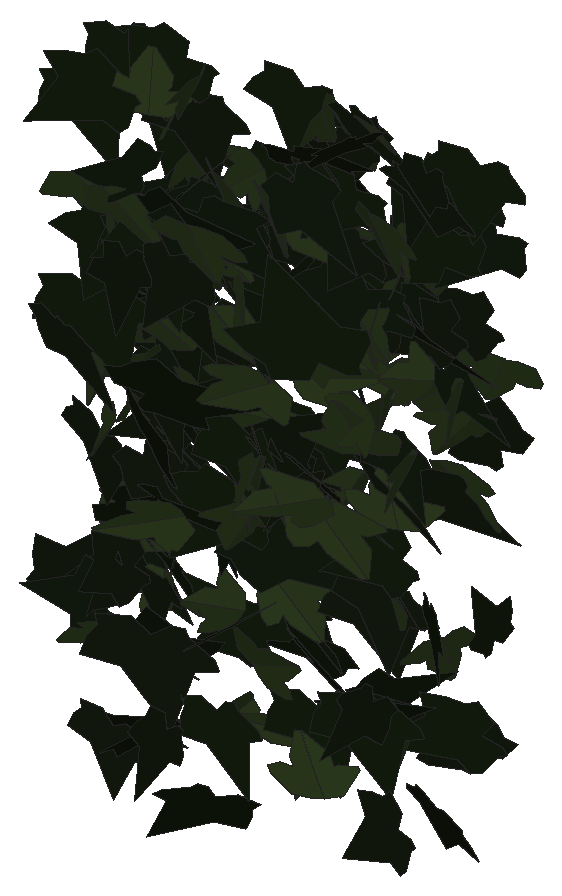
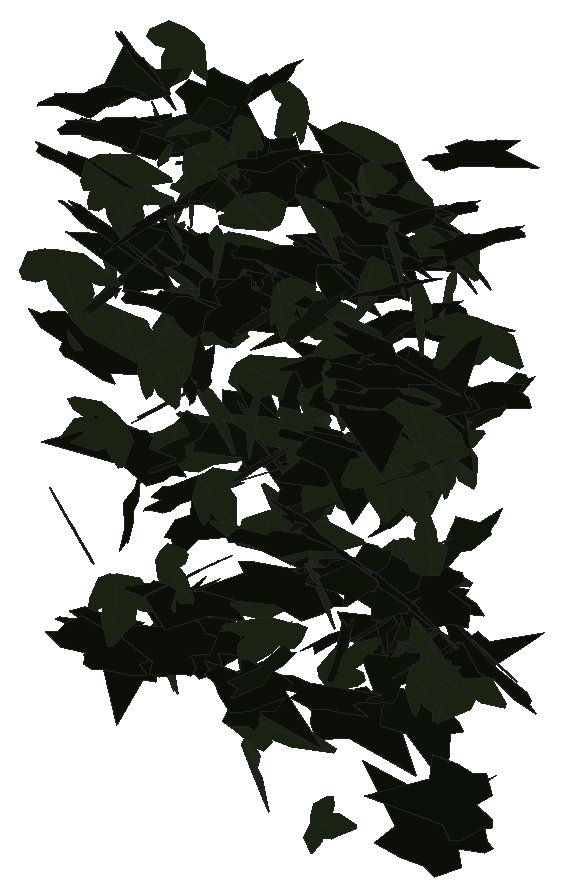
# SketchUp Ruby script. Lengths in millimetres.
U = 1.mm
M = Sketchup.active_model
def pt(a) = Geom::Point3d.new(a.map { |v| v * U })
def face(e, loops, mat)
  f = e.add_face(loops[0].map { |a| pt(a) })
  loops[1..].each { |l| e.add_face(l.map { |a| pt(a) }).erase! }
  f.material = f.back_material = mat if mat
  f
end
# faces: each face lists its corners as indices into pts; further lists are holes
def faces(e, pts, list, mat = nil) = list.each { |f| face(e, (f[0].is_a?(Array) ? f : [f]).map { |l| l.map { |i| pts[i] } }, mat) }
# xy, xz, yz: faces in a plane at the given z, y or x. An outline is a flat list of corners, or four numbers for a rectangle; further outlines are holes
def ring(l) = l.size == 4 ? [[l[0], l[1]], [l[2], l[1]], [l[2], l[3]], [l[0], l[3]]] : l.each_slice(2).to_a
def flat(e, list, mat, &to3) = list.each { |f| face(e, (f[0].is_a?(Array) ? f : [f]).map { |l| ring(l).map { |u, v| to3.(u, v) } }, mat) }
def xy(e, z, list, mat = nil) = flat(e, list, mat) { |x, y| [x, y, z] }
def xz(e, y, list, mat = nil) = flat(e, list, mat) { |x, z| [x, y, z] }
def yz(e, x, list, mat = nil) = flat(e, list, mat) { |y, z| [x, y, z] }
def lines(e, pts, list) = list.each { |a, b| e.add_line(pt(pts[a]), pt(pts[b])) }
# prism: a flat outline (further loops are holes) pulled along v
def prism(e, loops, v, mat = nil)
  f = face(e, loops, mat); d = Geom::Vector3d.new(v.map { |x| x * U })
  f.pushpull(f.normal.samedirection?(d) ? d.length : -d.length)
end
def box(e, o, s, mat = nil) = prism(e, [[o, [o[0] + s[0], o[1], o[2]], [o[0] + s[0], o[1] + s[1], o[2]], [o[0], o[1] + s[1], o[2]]]], [0, 0, s[2]], mat)
def at(x, y, z, deg = 0) = Geom::Transformation.translation(pt([x, y, z])) * Geom::Transformation.rotation(ORIGIN, Z_AXIS, deg.degrees)
def axes(o, x, y, z) = Geom::Transformation.new([*x, 0, *y, 0, *z, 0, *pt(o).to_a, 1])
def part(name) = M.definitions.add(name)
# library, detail: a bought-in or finely detailed component or shape, given as its bounding box
def library(name, o, s) = part(name).tap { |d| box(d.entities, o, s) }
def detail(e, o, s) = box(e.add_group.entities, o, s)
def put(e, d, t, mat = nil) = e.add_instance(d, t).tap { |i| i.material = mat if mat }
def group(e, t, mat = nil) = e.add_group.tap { |g| g.transformation = t; g.material = mat if mat }.entities
root = M.entities
M.materials.add("efeu1").color = [18, 25, 13]
M.materials.add("efeu2").color = [43, 57, 29]
c1 = part("ivyleaf_10")
p = [[0,12.8,-0.8],[-1.5,51.3,-10.9],[-4.9,51,-11.6],[-13.6,26.5,-7.3],[-13.2,15.9,-4.6],[-21.1,19.3,-7.2],
  [-29.5,16.3,-8.3],[-29.2,8.3,-6.2],[-19.7,-9.8,0.5],[-7.6,-13,4],[1,-12.2,5.8],[-0.4,51.1,-11.1],
  [-1.5,51.1,-10.9],[1,-12.4,5.9],[16.9,-12.4,3.5],[35.1,9.1,-5.1],[35,12.9,-6.1],[20.5,16.4,-4.9],
  [15.8,15,-3.8],[15.3,27.6,-7.1],[12.8,31.3,-7.8]]
faces(c1.entities,p,[[0,1,2,3,4,5,6,7,8,9,10],[11,12,0,13,14,15,16,17,18,19,20]],"efeu2")
c2 = part("ivyleaf_9")
p = [[39.1,54.8,31.7],[34.5,51.8,30.2],[-5.3,25.2,17.3],[-17.9,28.3,20.9],[-21.6,21.7,17],[-20.2,4.3,5.3],
  [-22.9,-0.3,2.5],[-17.1,-4,-0.6],[-2,-2.1,-1.2],[-0.7,-15.4,-10.1],[16.6,-22.3,-16.7],[21.1,-15.1,-12.5],
  [32.7,-10.7,-11],[46.1,-1.8,-6.6],[30.8,11.2,3.8]]
faces(c2.entities,p,[[0,1,2,3,4,5,6,7,8,9,10,11,12,13,14]],"efeu1")
put(root,c1,axes([4962,691.6,3292.7],[-1.7762,-0.47595,-0.52659],[1.00306,0.11802,-1.04073],[0.90488,-1.06506,0.11999]))
put(root,c1,axes([4979.1,780.1,2865.1],[-0.11101,-0.99344,0.61447],[0.34339,-0.61551,-0.978],[2.19648,0.04602,0.18395]))
put(root,c2,axes([4962.3,689.1,3419.8],[-0.22108,-1.1363,-0.36793],[0.15236,0.36143,-1.14149],[2.26804,-0.13504,0.04082]))
put(root,c2,axes([4939.4,733.4,2693.6],[1.88901,-0.45375,0.50394],[0.89286,-0.18557,-1.09108],[0.9319,1.09757,0.02386]))
put(root,c1,axes([4988.8,727.9,3151.3],[-0.03665,-1.1135,-0.2779],[0.06918,0.27721,-1.11324],[2.18311,-0.02748,0.03061]))
put(root,c2,axes([5005.5,726.8,3208.5],[1.06998,-1.00976,0.55],[-0.47547,0.49033,1.15558],[-2.13609,-0.61494,0.01828]))
put(root,c1,axes([4990.4,773.7,3212.6],[2.13036,-0.08977,-0.02516],[-0.04398,0.02656,-1.12268],[0.17189,1.11933,0.02462]))
put(root,c2,axes([4983.5,740.9,3469.3],[-0.04084,-1.09655,-0.41176],[0.17527,0.40897,-1.09393],[2.22233,-0.05241,0.07871]))
put(root,c2,axes([4997.7,622.6,2794.4],[-1.50185,0.96957,0.59516],[0.71509,-0.46156,1.25011],[2.04371,0.874,-0.00005]))
put(root,c1,axes([5003.9,735.5,2994.9],[-0.1621,-1.0748,-0.46005],[-0.09613,-0.45746,1.07809],[-2.223,0.09816,-0.01307]))
put(root,c2,axes([5040.4,775.6,2971.9],[-1.86084,0.45095,0.05619],[-0.09833,0.02213,-1.07672],[-0.85928,-0.97911,0.00154]))
put(root,c2,axes([5006,780.6,3125],[-0.72114,-0.87306,0.58255],[-0.01284,-0.61731,-0.92954],[1.99749,-0.31916,0.20434]))
put(root,c1,axes([4998.4,711.5,2839.6],[1.923,-0.60019,-0.2963],[0.54185,-0.10019,1.17382],[-1.15292,-1.04818,0.05746]))
put(root,c2,axes([5039.3,621.2,2794.9],[-0.3294,-0.12205,1.10477],[-1.64376,-0.68899,-0.21142],[1.3315,-0.88077,0.0123]))
put(root,c2,axes([4992.9,605.6,3152.4],[0.93684,-1.20241,0.03305],[0.03207,-0.02881,-1.29926],[2.28906,0.49251,0.00468]))
put(root,c2,axes([5006.1,668.5,2979.5],[-0.10325,-1.05962,0.85627],[0.02056,-0.85726,-1.06016],[2.59274,-0.0354,0.0425]))
put(root,c1,axes([5024.6,659.2,3099.4],[0.00047,-1.05884,0.61478],[0.35286,-0.60766,-1.04665],[2.30336,0.0933,0.16021]))
put(root,c2,axes([5045.9,630.4,3474.4],[-1.44899,-0.69541,0.66115],[-0.97674,-0.418,-1.03066],[1.54304,-0.91762,-0.03155]))
put(root,c1,axes([5031.4,763.2,3213.3],[1.65262,0.59442,-0.39867],[-0.66949,-0.19144,-1.05161],[-1.18631,0.93611,0.03809]))
put(root,c2,axes([5011.8,645.7,3180.4],[-0.7564,-1.09986,-0.64699],[0.36602,0.61827,-1.16919],[2.40083,-0.44078,-0.02559]))
put(root,c1,axes([5040.5,774.4,3118.5],[-1.57795,-0.74342,0.05772],[-0.04414,-0.06056,-1.1132],[1.41845,-0.8289,0.02956]))
put(root,c2,axes([5026.6,787.3,3370.4],[-0.81515,-1.03797,0.23762],[0.00907,-0.25799,-1.11836],[2.02656,-0.41636,0.10058]))
put(root,c2,axes([5037.8,662.7,3261.3],[-1.41165,-0.90871,0.06733],[-0.07959,-0.05278,-1.17299],[1.73236,-0.7429,0.00098]))
put(root,c2,axes([5053,682.6,3175.3],[0.27885,0.87061,-0.72867],[-0.44657,-0.69563,-0.87832],[-2.11407,0.26178,0.08942]))
put(root,c2,axes([5057.8,752,3462.3],[-2.05843,-0.38687,0.23688],[-0.32979,-0.21366,-1.14012],[0.79788,-1.08639,0.13988]))
put(root,c1,axes([5012.7,770.2,3111.9],[-1.41196,0.24976,-0.81706],[1.29856,-0.4781,-0.76567],[-0.97868,-0.99469,0.16286]))
put(root,c1,axes([5051.1,739.7,3405.5],[0.62617,-0.90558,-0.61868],[-0.30653,0.59902,-0.96246],[2.06469,0.36358,0.04474]))
put(root,c2,axes([5050.8,787.2,3220.5],[-1.62125,-0.73929,0.04152],[-0.09269,-0.00721,-1.12761],[1.40617,-0.85284,-0.02646]))
put(root,c1,axes([5050,686.3,3089.8],[-0.47019,-1.12116,-0.09841],[0.04239,0.09586,-1.14806],[2.14159,-0.24805,0.00112]))
put(root,c2,axes([5087.7,766.2,3273.2],[-1.70987,0.32367,0.60945],[-1.10847,0.18092,-0.95467],[-0.70437,-1.07044,0.02293]))
put(root,c1,axes([5041.3,707.7,3421.9],[1.38267,0.90655,-0.29073],[0.33671,0.23079,1.16172],[1.78034,-0.74771,0.00608]))
put(root,c2,axes([5027,773.3,2927.3],[0.58754,-1.07262,-0.19886],[-0.14997,0.1842,-1.1159],[2.07078,0.31768,-0.02439]))
put(root,c2,axes([5056.4,785.9,3250.7],[-1.64631,-0.70667,-0.02188],[0.00764,0.02966,-1.1168],[1.34556,-0.86479,-0.02043]))
put(root,c2,axes([5010.6,677.5,2589.3],[2.08269,0.63073,-0.20183],[0.32875,0.10447,1.26306],[1.21673,-1.10785,0.0042]))
put(root,c2,axes([5087.8,618.5,2857],[-2.0039,0.61637,0.0026],[-0.01113,-0.00483,-1.22004],[-1.17303,-1.0529,0.00712]))
put(root,c1,axes([5052.6,610.6,2766.9],[-1.38708,-0.74622,-0.42917],[0.61993,0.28146,-1.04254],[1.51652,-0.79758,0.03363]))
put(root,c2,axes([5069.1,761.8,3202.7],[1.36679,0.57725,-0.66021],[-1.18936,-0.26183,-0.90871],[-1.17098,0.93971,0.15236]))
put(root,c2,axes([5038.9,685.2,2831.7],[0.78028,-0.90524,-0.67299],[-0.37695,0.64717,-0.99117],[2.11345,0.44964,0.07169]))
put(root,c2,axes([5048,634.8,2621],[-0.27849,-1.08269,0.32411],[-0.05162,-0.32336,-1.09242],[2.1503,-0.14798,0.01575]))
put(root,c1,axes([5067.9,611.8,3277.5],[0.37153,-0.41456,-1.18221],[-0.03147,1.19552,-0.42196],[2.38411,0.08039,0.17866]))
put(root,c2,axes([5026.8,756,2952.5],[1.24593,-0.75717,0.41916],[0.56491,-0.29726,-1.00055],[1.54722,0.71826,0.02777]))
put(root,c2,axes([5096.4,622.9,3378.1],[-1.13024,0.95216,0.26363],[-0.33065,0.20215,-1.12148],[-1.85102,-0.6175,0.03936]))
put(root,c2,axes([5045.3,724.2,3037],[0.25384,-1.12104,0.29146],[-0.01109,-0.29403,-1.12827],[2.20447,0.1276,-0.03923]))
put(root,c2,axes([5092.9,698.4,3204.6],[-2.16324,0.1888,-0.00332],[0.00692,0.00163,-1.1522],[-0.3593,-1.13664,-0.00221]))
put(root,c2,axes([5056.6,707.2,3086.5],[0.71742,-0.84749,-0.6327],[-0.44905,0.58737,-0.92735],[1.96212,0.4443,0.0191]))
put(root,c1,axes([5083.3,656.5,3282.1],[0.95168,-0.76891,-0.81576],[-0.27783,0.84097,-0.88215],[2.11536,0.45638,0.25114]))
put(root,c2,axes([5053,733.4,3272.6],[0.88155,-1.02496,-0.33515],[-0.12914,0.33633,-1.12236],[2.04827,0.46233,0.07348]))
put(root,c1,axes([5063.1,723.2,3119],[-1.66927,-0.36223,-0.60321],[1.06161,0.22962,-0.94894],[0.81624,-1.03943,0.00058]))
put(root,c2,axes([5049.2,730.4,2814.6],[0.49849,-0.88321,0.69389],[0.34991,-0.66918,-0.92116],[2.10881,0.31982,-0.01118]))
put(root,c2,axes([5059.9,683.2,2961.8],[0.69056,-0.99249,-0.57538],[-0.15577,0.57954,-1.05128],[2.17782,0.35616,0.10725]))
put(root,c1,axes([5082.3,734.6,3350],[-0.06694,-0.94096,-0.68531],[0.4226,0.66761,-0.92805],[2.17477,-0.15869,0.15925]))
put(root,c1,axes([5095.1,566.1,3070.7],[0.48781,-1.15549,-0.39899],[-0.18163,0.38751,-1.18355],[2.31944,0.27336,-0.00877]))
put(root,c2,axes([5043.5,657.6,2907.7],[1.0219,0.47109,-1.0485],[1.15049,0.86857,0.69981],[1.86071,-0.79576,0.14313]))
put(root,c1,axes([5071.4,611.5,3343.4],[-1.84166,0.15036,-0.60938],[1.12188,-0.16694,-0.97724],[-0.41032,-1.13131,0.06321]))
put(root,c1,axes([5118.3,648.2,2916.5],[0.62578,0.34799,-1.06473],[-1.76212,-0.54014,-0.46246],[-1.19993,0.97468,0.12386]))
put(root,c2,axes([5062.7,765.8,2968.6],[1.25445,-0.92377,0.09274],[0.10943,-0.0729,-1.1348],[1.76356,0.66162,0.00445]))
put(root,c2,axes([5075.6,668.9,3268.8],[-0.3092,-1.28596,-0.40789],[0.05981,0.40712,-1.29604],[2.56691,-0.16439,-0.01893]))
put(root,c2,axes([5100.2,751,3114.2],[0.87271,0.9838,-0.15027],[-0.19445,-0.11805,-1.08459],[-1.88408,0.46788,0.04233]))
put(root,c1,axes([5099.2,722.6,3460],[0.1377,-1.17115,-0.05305],[-0.00766,0.05291,-1.17338],[2.23121,0.07246,-0.00075]))
put(root,c1,axes([5089.2,670.1,2813.4],[-0.40099,-0.89114,0.74896],[0.77744,-0.76932,-0.80046],[2.07457,0.11606,0.44473]))
put(root,c2,axes([5082.6,660.8,2832.3],[-0.06177,-0.91861,0.56879],[0.1299,-0.56965,-0.91611],[2.0522,0.00841,0.07511]))
put(root,c2,axes([5089.6,738.9,3416.9],[-1.30282,-0.45883,-0.79864],[1.49916,0.22408,-0.8039],[0.90852,-1.02772,0.18128]))
put(root,c2,axes([5128.2,647.8,3307.6],[-1.57122,-0.55631,0.63998],[-0.7603,-0.53271,-0.97839],[1.42354,-0.89853,0.18382]))
put(root,c2,axes([5099.1,703.3,2882.7],[-0.55172,0.08558,-1.09684],[1.62892,-0.69515,-0.28045],[-1.31562,-0.89658,0.11275]))
put(root,c1,axes([5117,760.3,3214.2],[-0.15948,-1.13176,-0.31469],[0.00378,0.31535,-1.13467],[2.23567,-0.08126,-0.02053]))
put(root,c2,axes([5086.3,688.5,3208.6],[-0.93128,-0.2087,-1.06709],[1.91205,0.36075,-0.53125],[0.79142,-1.11713,0.0278]))
put(root,c2,axes([5080.9,733.5,3095.9],[-0.44193,-0.39322,-1.34017],[1.84259,0.93388,-0.44176],[1.91587,-0.98886,0.11573]))
put(root,c1,axes([5106,700.1,3071.7],[-1.11708,0.82154,-0.63829],[0.65941,-0.53667,-1.00935],[-1.86697,-0.68111,0.02541]))
put(root,c2,axes([5103.7,769.2,2848.1],[0.5471,-0.43677,-1.01931],[1.5509,-0.63099,0.50019],[-1.43146,-0.85057,0.15235]))
put(root,c1,axes([5135.4,774.4,2617.8],[0.06732,0.44837,-0.96186],[-0.74895,-0.88824,-0.42852],[-1.87574,0.37075,0.13658]))
put(root,c2,axes([5123.2,564.5,3300.4],[-1.3524,0.00722,-0.91749],[1.69872,-0.26338,-0.69336],[-0.4045,-1.1302,0.15572]))
put(root,c2,axes([5148.6,569.5,2677.1],[-0.01569,1.12461,-0.17765],[0.01623,-0.17759,-1.12462],[-2.16684,-0.00947,-0.00714]))
put(root,c2,axes([5146.2,768.5,3123.9],[-1.82036,-0.53684,0.00004],[0.13727,-0.12859,-1.08688],[1.01245,-0.94779,0.14744]))
put(root,c1,axes([5124.9,724.1,3249.9],[-1.1355,-0.74729,-0.61186],[0.98134,0.36167,-0.94451],[1.55427,-0.77429,0.14934]))
put(root,c2,axes([5124.4,762.4,3230.2],[-0.44947,-1.04544,-0.38737],[0.20443,0.37278,-1.07158],[2.11201,-0.25857,0.02129]))
put(root,c2,axes([5143.1,603.6,2766.9],[1.78008,0.28135,0.78223],[-1.43266,-0.21291,0.97666],[0.67123,-1.20056,0.01012]))
put(root,c2,axes([5127.3,669.7,3345.4],[0.573,1.11029,0.52357],[-0.32187,-0.49643,1.14998],[2.31398,-0.34399,0.03031]))
put(root,c2,axes([5158.9,719.7,2923.2],[-1.53721,-0.88905,0.38187],[-0.49566,-0.27932,-1.20115],[1.77357,-0.84863,-0.0047]))
put(root,c2,axes([5188.1,754.6,2994.8],[-1.27873,0.58417,0.59683],[-0.93659,0.34196,-0.8887],[-1.28419,-0.83109,0.05385]))
put(root,c2,axes([5128.8,603.8,3044.5],[-0.31569,-0.07296,1.41238],[0.25482,-1.41648,-0.05745],[2.67953,0.12611,0.17186]))
put(root,c1,axes([5157.5,713.1,2785.7],[-0.02756,0.54847,1.09855],[0.08283,-1.0977,0.54862],[2.33538,0.04541,-0.00649]))
put(root,c2,axes([5192.7,731.2,2750.9],[-1.77075,-0.51547,-0.35197],[-0.58667,-0.16989,1.06365],[-1.03295,0.98014,-0.00074]))
put(root,c1,axes([5158.4,732.9,3047.7],[-1.90168,0.52266,0.0024],[-0.00411,0.00105,-1.12764],[-0.99472,-0.99921,0.00007]))
put(root,c1,axes([5165.8,741.7,2922.3],[0.9421,-0.99677,-0.19402],[-0.19543,0.1656,-1.11277],[1.92275,0.50522,-0.01804]))
put(root,c2,axes([5137.2,644,3302.9],[0.21154,1.07817,-0.5978],[0.1349,0.59364,1.08385],[2.3424,-0.13156,-0.00844]))
put(root,c2,axes([5167.2,698.7,3327],[-1.91663,-0.31467,-0.45748],[0.84289,0.11626,-1.0549],[0.63738,-1.09997,0.01937]))
put(root,c2,axes([5143.7,751.1,3021.8],[0.58821,-1.08031,0.19513],[0.13591,-0.1825,-1.12351],[2.0849,0.31668,0.01819]))
put(root,c1,axes([5157.5,699.5,3178],[-1.75806,-0.40249,-0.4536],[0.95304,-0.04007,-0.98421],[0.65097,-1.02832,0.2159]))
put(root,c2,axes([5148,750.6,3275.3],[1.30192,-0.93214,-0.41267],[-0.2554,0.41031,-1.14925],[1.92325,0.68549,0.12674]))
put(root,c2,axes([5126.2,606.6,3104.4],[0.63751,-0.13995,1.31842],[2.46214,-0.26313,-0.35661],[0.55227,1.33462,0.06795]))
put(root,c2,axes([5191.5,686.4,3305.6],[-1.00075,0.60273,-0.83521],[0.82742,-0.72025,-0.79347],[-1.77707,-0.67477,0.1009]))
put(root,c2,axes([5190.5,595.4,3304.6],[-2.0816,0.15367,-0.54522],[1.02796,-0.07441,-1.10448],[-0.32494,-1.21983,-0.00131]))
put(root,c1,axes([5195.5,708.6,3379.9],[1.23356,-0.75709,-0.57442],[-0.66998,0.45457,-0.99634],[1.68003,0.73717,0.02444]))
put(root,c2,axes([5170.1,554.9,2818.8],[-1.22925,-0.99792,-0.6463],[0.5967,0.56652,-1.18806],[2.18268,-0.71689,-0.03919]))
put(root,c1,axes([5187.4,660.8,3384.8],[-1.50168,0.82604,0.16505],[-0.19031,0.1327,-1.14217],[-1.59186,-0.79511,-0.01915]))
put(root,c1,axes([5185.4,775.9,3300.6],[-0.02164,-1.11273,0.11096],[0.48164,-0.11065,-1.08366],[2.07303,0.01409,0.25293]))
put(root,c1,axes([5206,693.6,2936.5],[-0.98783,-0.99487,0.25396],[-0.24447,-0.21941,-1.12206],[1.93879,-0.53456,-0.01209]))
put(root,c2,axes([5199.6,783,2979.3],[-1.60428,-0.7139,-0.09737],[0.14479,0.06083,-1.10462],[1.36361,-0.84636,0.00274]))
put(root,c2,axes([5202,772.1,3352.1],[-1.64883,-0.7284,-0.03226],[0.05187,0.01771,-1.13186],[1.38669,-0.86676,0.00398]))
put(root,c2,axes([5174.6,595.3,3347.8],[0.0335,-0.21691,1.21306],[1.57166,-0.8984,-0.17263],[1.7408,0.81529,0.13251]))
put(root,c2,axes([5258.4,756,2760.3],[0.12386,0.22115,-1.08745],[-1.89327,-0.47113,-0.15535],[-0.93598,0.98225,0.17033]))
put(root,c2,axes([5203.2,775.8,3268.7],[0.5977,-1.09555,-0.11039],[-0.04543,0.10799,-1.13966],[2.09512,0.31488,0.00678]))
put(root,c1,axes([5224.9,759.5,2948.9],[2.03409,0.30106,0.07668],[-0.16111,0.0179,1.10964],[0.56889,-1.07137,0.04008]))
put(root,c2,axes([5221.6,771.7,3468.5],[-0.79367,-1.09053,0.07911],[0.03653,-0.09196,-1.16644],[2.08063,-0.41438,0.05066]))
put(root,c2,axes([5205.7,778.9,2793.8],[0.67868,-1.08529,0.1425],[0.10741,-0.13144,-1.1423],[2.08048,0.36082,0.01249]))
put(root,c2,axes([5216.2,677.8,3046],[-0.47912,-1.27421,-0.24221],[0.13157,0.2332,-1.29865],[2.46499,-0.26011,0.02224]))
put(root,c1,axes([5244,756,3120.8],[-0.59578,0.98969,0.36686],[-0.5765,0.28232,-1.0201],[-1.92432,-0.39099,0.19203]))
put(root,c2,axes([5258.8,557.1,2635.5],[0.26361,0.63063,-0.96191],[-0.45954,-0.93133,-0.64534],[-2.14029,0.27764,0.02009]))
put(root,c2,axes([5211.1,596.7,3375.8],[-0.2919,-0.45833,-1.19075],[0.87058,1.09985,-0.48225],[2.2669,-0.4814,0.03188]))
put(root,c2,axes([5204.1,700.4,3007.4],[0.71887,-0.59464,0.91033],[0.83586,-0.79815,-0.70359],[1.8931,0.57821,-0.03502]))
put(root,c1,axes([5241.3,547.6,3382.1],[-2.21019,0.09247,-0.14215],[0.27003,-0.00898,-1.16497],[-0.17676,-1.16993,-0.00229]))
put(root,c2,axes([5201.1,723.3,2887.6],[0.62385,-0.4149,-1.23904],[0.9439,1.22135,-0.27777],[2.30075,-0.38856,0.44992]))
put(root,c1,axes([5227.9,731.1,2822.2],[0.95109,0.9962,0.5115],[0.3802,0.47184,-1.11411],[-2.0971,0.53734,0.03]))
put(root,c1,axes([5201.2,697.2,3067.6],[-0.17291,0.0383,-1.23942],[2.35747,0.06027,-0.08894],[0.10913,-1.24128,-0.04256]))
put(root,c2,axes([5248.8,481.2,2754.2],[-1.60022,0.2738,-0.77264],[1.36469,-0.29065,-0.88331],[-0.75596,-1.10428,0.04092]))
put(root,c1,axes([5293.8,699,2669.6],[0.47923,-0.03689,-1.16536],[-2.21836,0.02133,-0.25253],[0.05451,1.19206,-0.03154]))
put(root,c2,axes([5233.3,685.6,3027.2],[-1.00488,0.57376,0.97393],[1.27358,-0.70767,0.77969],[1.73383,0.85236,-0.00826]))
put(root,c2,axes([5267.7,781.1,3260.3],[-0.37189,-0.28508,-1.11096],[0.76624,-1.0723,0.20435],[-2.04398,-0.35011,0.27874]))
put(root,c2,axes([5249.3,772.3,3031.3],[-0.35901,-1.08534,0.18352],[0.14754,-0.19883,-1.09621],[2.08974,-0.17242,0.10892]))
put(root,c2,axes([5233,761.6,2730.4],[0.51917,-0.67801,0.87201],[0.71962,-0.78663,-0.72991],[1.97524,0.4648,0.03672]))
put(root,c1,axes([5290.1,602.6,3174.5],[1.60785,0.18006,-0.76482],[-1.4854,0.06261,-0.84736],[-0.1727,1.13787,0.16765]))
put(root,c1,axes([5258.7,620.7,3040.8],[0.37603,-0.42515,1.06104],[0.90692,-0.9481,-0.46863],[1.97738,0.51569,0.01316]))
put(root,c2,axes([5256.7,569.2,2741.3],[0.12193,-1.19728,-0.16457],[-0.05748,0.16316,-1.1988],[2.29936,0.06757,-0.02124]))
put(root,c1,axes([5276.3,737.1,3470.9],[0.01436,-0.99563,-0.59524],[0.35412,0.58859,-0.98213],[2.17911,-0.08909,0.16352]))
put(root,c1,axes([5284.6,710.4,2623.1],[0.84878,-1.02818,-0.13222],[-0.08675,0.12435,-1.12071],[1.97103,0.44823,0.00761]))
put(root,c2,axes([5263.4,723.1,3023],[-0.03161,-1.06986,0.41077],[0.04014,-0.41103,-1.06968],[2.1807,-0.00794,0.02565]))
put(root,c1,axes([5281,773.7,3330.1],[-0.86752,1.04116,-0.13566],[-0.21171,-0.19495,-1.12242],[-1.98704,-0.43379,0.17882]))
put(root,c2,axes([5298.8,780.1,3260],[-0.03767,0.05104,-1.25533],[0.01933,-1.25544,-0.05121],[-2.39104,-0.01095,0.01936]))
put(root,c1,axes([5259.8,605.3,3282],[0.2393,-0.34975,1.10376],[1.34334,-0.85695,-0.35195],[1.74682,0.70692,0.11945]))
put(root,c2,axes([5329.6,646.5,3224],[-1.5607,0.10315,-0.88856],[-1.69986,-0.02771,0.82107],[0.09422,1.20882,0.09464]))
put(root,c2,axes([5264.3,710.2,3426.7],[2.08805,0.40483,0.1263],[0.21954,0.05221,-1.1694],[-0.77666,1.10314,0.009]))
put(root,c1,axes([5277.9,617.1,3052.6],[0.8028,-0.95085,0.69676],[0.7923,-0.57218,-1.03287],[2.09894,0.57966,0.12339]))
put(root,c2,axes([5323.6,759.2,3435.9],[-1.72457,0.71886,-0.01641],[0.01869,-0.01402,-1.15665],[-1.36837,-0.90618,0.00488]))
put(root,c2,axes([5269,750.5,3418.5],[1.53769,-0.93243,-0.22441],[-0.2763,0.17114,-1.23378],[1.80424,0.82089,0.00232]))
put(root,c2,axes([5285,629.7,3229.1],[0.6708,-0.39534,-1.02793],[-0.62031,0.9935,-0.49386],[2.00216,0.44026,0.19139]))
put(root,c1,axes([5304.6,765.3,3456.6],[-1.98468,0.49449,-0.00391],[0.00667,-0.00174,-1.15412],[-0.94112,-1.04282,0.00007]))
put(root,c2,axes([5313.6,668.9,3036.2],[-1.49582,0.35453,-0.68866],[1.03391,-0.44703,-0.85013],[-1.05079,-0.94453,0.14386]))
put(root,c2,axes([5315.7,602.8,3034],[0.41481,-0.84489,0.75376],[0.18019,0.77851,0.84526],[-2.14736,-0.09789,0.21653]))
put(root,c1,axes([5311.1,754.3,2990.4],[-0.21368,-1.01517,0.57829],[0.167,-0.58665,-1.01279],[2.21728,-0.05365,0.13201]))
put(root,c1,axes([5308.6,596.2,3430.6],[-1.32275,0.87875,-0.32007],[0.26072,-0.29883,-1.11787],[-1.76073,-0.70441,0.07493]))
put(root,c1,axes([5287.4,690.1,3340.5],[-0.37172,-0.12717,1.20138],[1.69603,0.80652,0.23025],[-1.55241,0.91159,-0.03611]))
put(root,c1,axes([5335.9,730.4,3095.4],[1.29342,-0.81501,-0.49024],[-0.58338,0.3827,-1.06114],[1.71354,0.74548,0.00878]))
put(root,c2,axes([5304,482.7,2893.5],[0.54639,1.13795,0.14114],[-0.06603,-0.13681,1.1736],[2.18134,-0.28918,0.00018]))
put(root,c2,axes([5298,672.9,3038.2],[2.09342,-0.65109,0.07127],[0.13686,-0.01841,-1.27803],[1.23902,1.1021,0.02075]))
put(root,c2,axes([5354.9,698.6,3480.1],[-0.65108,0.84605,-0.72768],[0.15429,-0.74025,-0.89878],[-2.11824,-0.31397,0.1582]))
put(root,c2,axes([5340.9,715.2,3401.3],[-1.40892,-0.78602,0.47071],[-0.21259,-0.52322,-1.04938],[1.73067,-0.70416,0.2543]))
put(root,c1,axes([5338.4,625.3,3236.4],[-2.3422,-0.17092,-0.1005],[0.19066,0.0093,-1.24247],[0.32566,-1.23473,0.00456]))
put(root,c1,axes([5367.5,595.8,3053.9],[-0.84664,-0.28803,1.0474],[-1.24973,-0.83032,-0.50722],[1.64692,-0.77814,0.15355]))
put(root,c2,axes([5356.3,789.4,3244.3],[-1.78069,-0.64753,0.04356],[-0.01309,-0.06652,-1.13672],[1.2351,-0.93428,0.05075]))
put(root,c2,axes([5312.3,756.2,3470.3],[1.11753,-0.98945,0.09964],[0.40067,0.01059,-1.13547],[1.84976,0.59548,0.18575]))
put(root,c1,axes([5324.9,562.6,2832.8],[-1.38844,0.19166,0.88927],[1.62347,-0.25191,0.75409],[0.60151,1.1223,0.0174]))
put(root,c2,axes([5372.4,723.4,3247.6],[-2.0994,0.18462,-0.26502],[0.49478,-0.05214,-1.11841],[-0.36478,-1.13328,0.00828]))
put(root,c2,axes([5340.9,647.6,2742.8],[-0.42576,-1.16651,-0.38425],[0.08331,0.38275,-1.18744],[2.33596,-0.22626,-0.02768]))
put(root,c1,axes([5381.8,743,2854.8],[0.10383,0.10617,-1.23968],[-1.06122,1.11137,0.07064],[2.11688,0.55194,0.09622]))
put(root,c2,axes([5341.6,736.7,3110.4],[-0.03914,-0.26072,1.14438],[-0.08702,-1.14351,-0.26134],[2.2321,-0.04915,0.00988]))
put(root,c2,axes([5344.8,760.3,2841.2],[-1.17997,-0.76027,-0.60995],[0.78966,0.44826,-0.98048],[1.67859,-0.74531,0.03248]))
put(root,c2,axes([5359.9,701.1,3350.5],[-0.65771,-0.87945,0.61497],[-0.34948,-0.58808,-0.94419],[2.01226,-0.38958,0.03702]))
put(root,c2,axes([5368.1,705.2,3281.6],[-2.19118,-0.41076,-0.45317],[0.80874,0.15754,-1.22238],[0.83722,-1.22722,-0.00524]))
put(root,c2,axes([5344.5,605.8,3457.6],[0.70905,-1.10985,-0.79003],[-0.51476,0.74248,-1.17059],[2.54115,0.46008,-0.01669]))
put(root,c1,axes([5368.8,782.2,3146.9],[-0.30289,-1.06257,0.40838],[0.09267,-0.41832,-1.06948],[2.16452,-0.13078,0.10293]))
put(root,c2,axes([5350.8,755.4,2858.5],[-0.24188,-1.28295,0.25424],[-0.07422,-0.25161,-1.28916],[2.48809,-0.13223,-0.01374]))
put(root,c1,axes([5349.7,632.5,3190.4],[0.00604,-0.0802,1.18514],[0.73611,1.12063,0.0748],[-2.13753,0.38569,0.02911]))
put(root,c1,axes([5335.9,711.4,3187.4],[1.37229,0.22948,0.8938],[1.56903,0.34942,-0.75478],[-0.78903,1.09394,0.05359]))
put(root,c1,axes([5348,650,2997.4],[1.87082,0.42679,0.65811],[1.15405,0.25584,-1.07162],[-0.94695,1.15495,-0.00581]))
put(root,c2,axes([5402.9,721.3,2931.2],[-0.88456,-0.43933,0.94732],[-1.22285,-0.69708,-0.63851],[1.56664,-0.79216,0.03649]))
put(root,c1,axes([5397.1,695.1,3151],[-0.38926,-1.11241,-0.40418],[0.0633,0.40461,-1.13041],[2.25166,-0.20369,-0.03809]))
put(root,c2,axes([5362.7,738.6,3022.9],[0.99789,-0.9878,0.25663],[0.28895,-0.20981,-1.11779],[1.92078,0.54475,0.03483]))
put(root,c2,axes([5373.6,748.7,3338.8],[0.80419,-0.90025,-0.75192],[-0.37197,0.73401,-0.98864],[2.20116,0.45294,0.10764]))
put(root,c2,axes([5358.8,685.8,2729.6],[1.86603,0.49921,-0.2946],[0.43228,0.20171,1.09774],[1.01497,-1.0037,0.07409]))
put(root,c1,axes([5395.1,723.5,2987],[1.68916,0.7181,0.02468],[-0.046,-0.00937,1.14164],[1.36673,-0.88783,0.00792]))
put(root,c2,axes([5371.1,719.2,2734.6],[0.17851,-0.01048,1.07761],[1.80971,0.50983,-0.0778],[-0.96517,0.954,0.05342]))
put(root,c2,axes([5423.7,543,3284.4],[-2.58902,-0.41519,0.29721],[0.55085,0.06974,1.42219],[-0.80057,1.39069,0.01741]))
put(root,c1,axes([5398.1,721.1,3307.9],[0.94174,-0.99019,0.21228],[0.16762,-0.19329,-1.10692],[1.92005,0.50254,-0.00749]))
put(root,c2,axes([5380.8,734.2,3074.2],[0.32674,-1.15824,-0.04517],[-0.01255,0.04468,-1.17089],[2.206,0.1718,0.00003]))
put(root,c2,axes([5396.7,760.2,3276.3],[1.08837,-0.50748,-0.82242],[-0.78493,0.73606,-0.74097],[1.66332,0.67942,0.18847]))
put(root,c1,axes([5414,557,2710.5],[1.24564,0.96806,0.06775],[-0.09991,-0.04628,1.16842],[1.84422,-0.65636,0.01754]))
put(root,c1,axes([5432.4,745.2,3154.4],[1.27829,-0.54951,-0.7788],[-0.63232,0.75801,-0.82137],[1.70026,0.69503,0.28006]))
put(root,c1,axes([5438.3,768.6,3377.6],[-1.38761,-0.87195,0.16764],[-0.21026,-0.12615,-1.1366],[1.67675,-0.73741,-0.00379]))
put(root,c1,axes([5446.2,599.4,3153.6],[-1.95965,-0.39652,-0.41797],[-0.74564,-0.1457,1.10336],[-0.80393,1.10167,-0.00452]))
put(root,c2,axes([5417.9,643.4,2768.8],[-0.64016,-1.09173,-0.47699],[0.24622,0.45923,-1.14232],[2.25403,-0.36022,-0.01069]))
put(root,c1,axes([5453.9,609.7,3291.1],[-0.27411,0.49585,1.05803],[-1.22347,0.85657,-0.48894],[-1.85699,-0.63754,0.16596]))
put(root,c1,axes([5432.3,690.1,2702.8],[0.8104,-1.02587,0.36752],[0.3518,-0.32086,-1.1098],[2.04388,0.46198,0.0453]))
put(root,c1,axes([5438.4,762.5,2815.5],[-0.82494,-1.11619,-0.35215],[0.30678,0.31501,-1.1969],[2.20633,-0.46114,0.03476]))
put(root,c1,axes([5446.8,591.4,3193.1],[1.45974,-0.80704,-0.3962],[-0.52896,0.28244,-1.11335],[1.62726,0.81577,-0.00649]))
put(root,c2,axes([5469.9,728,3255.4],[-1.91279,0.46839,0.08214],[-0.13459,0.04271,-1.10879],[-0.89497,-1.00749,-0.00882]))
put(root,c2,axes([5402.5,759,3014.6],[0.30968,-0.19362,-1.10253],[1.52741,0.79686,-0.0215],[1.4852,-0.77914,0.252]))
put(root,c1,axes([5451.8,746.7,3336.6],[-1.06089,-0.98208,-0.02114],[0.01228,0.02064,-1.12924],[1.86948,-0.55744,-0.00458]))
put(root,c1,axes([5447.3,614.4,3296.8],[-0.42283,0.99219,0.58733],[-0.42799,0.54936,-1.01311],[-2.15224,-0.30417,0.08608]))
put(root,c1,axes([5445.4,684.2,3090.4],[0.51967,-1.12127,0.43947],[0.23983,-0.42155,-1.15384],[2.27948,0.29998,0.02121]))
put(root,c2,axes([5406.8,725.3,3240],[1.22054,-0.62728,0.72208],[1.14189,-0.41324,-0.89186],[1.41774,0.87288,0.09669]))
put(root,c1,axes([5436.3,682.5,3379.6],[-0.18673,0.15125,-1.11877],[0.60753,-1.07344,-0.17311],[-2.06093,-0.33014,0.05033]))
put(root,c2,axes([5461.4,768.1,3428.4],[-1.37431,-0.9,0.04438],[-0.05217,-0.0349,-1.15388],[1.71418,-0.72262,0.00046]))
put(root,c2,axes([5499.1,739.6,2702.1],[-0.06507,0.10625,1.16073],[-2.21628,0.04688,-0.03859],[-0.0955,-1.16028,0.10473]))
put(root,c2,axes([5487.4,697.3,3365.6],[-2.16412,-0.42775,0.18167],[0.37188,-0.00435,1.21275],[-0.8025,1.15151,0.07207]))
put(root,c1,axes([5443.6,773.7,3036],[-1.48462,0.51311,-0.68013],[1.10604,-0.35385,-0.9335],[-1.18569,-0.97256,-0.01919]))
put(root,c1,axes([5467.7,679.2,3213],[-0.0594,0.45651,1.088],[0.22922,-1.08147,0.45722],[2.23385,0.12311,-0.01798]))
put(root,c2,axes([5471.3,585,2823.9],[-0.04528,0.07537,-1.1814],[0.90519,-1.08146,-0.07857],[-2.06317,-0.47614,-0.00854]))
put(root,c1,axes([5473.1,597.4,3456.1],[-1.82909,0.69561,-0.02515],[0.03952,-0.0142,-1.18639],[-1.32416,-0.96129,-0.00068]))
put(root,c2,axes([5469,687.4,3478.2],[-1.49279,0.16839,-0.8535],[1.56334,-0.23508,-0.80127],[-0.54523,-1.13509,0.03933]))
put(root,c1,axes([5492.8,738.5,3141],[-1.0453,-0.90116,0.43278],[-0.46125,-0.35904,-1.05518],[1.84587,-0.60004,-0.01859]))
put(root,c2,axes([5513.1,729.6,2733.7],[-1.85285,-0.15093,0.56477],[-1.05973,-0.09474,-0.98515],[0.33887,-1.12151,0.00722]))
put(root,c2,axes([5522.5,753.9,3110.2],[-0.53858,0.30456,1.14676],[-1.60757,0.77623,-0.41459],[-1.58589,-0.89027,0.03081]))
put(root,c2,axes([5461.4,708,3442.6],[-0.65781,-0.82107,0.78571],[0.64196,-0.85835,-0.7486],[2.0654,0.00529,0.48292]))
put(root,c2,axes([5513.1,737.1,3277],[-1.97405,0.38549,0.13701],[-0.23173,0.06563,-1.10639],[-0.74335,-1.04418,-0.01896]))
put(root,c2,axes([5461.9,707.1,2886.4],[0.19412,-0.03313,-1.17115],[1.83168,-0.66805,0.10272],[-1.27164,-0.96732,-0.03082]))
put(root,c2,axes([5464.6,736.6,3193.6],[1.14105,-0.85816,-0.52457],[-0.4107,0.48672,-1.04288],[1.86963,0.63066,0.09106]))
put(root,c2,axes([5500.4,775.8,3372.4],[-2.12335,-0.20178,-0.20387],[0.40758,-0.04129,-1.13112],[0.36317,-1.1334,0.0775]))
put(root,c2,axes([5485,767.9,3458.9],[-0.88403,-1.06379,-0.0732],[0.06444,0.06509,-1.16077],[2.02837,-0.4657,0.00497]))
put(root,c2,axes([5511.1,656.8,2665.4],[1.53914,-0.07015,-0.84859],[-1.59545,0.13956,-0.81044],[0.28407,1.16389,0.04603]))
put(root,c2,axes([5529.2,740.4,2864.5],[-0.18656,0.52806,0.95927],[-0.25552,0.95004,-0.5367],[-2.0683,-0.165,-0.02022]))
put(root,c1,axes([5526.1,759.3,3215.9],[-1.87204,-0.48084,0.23605],[-0.39641,-0.11138,-1.09483],[0.93922,-1.0054,0.0084]))
put(root,c2,axes([5516.1,574.8,2676.3],[-0.54216,-0.62266,1.06046],[-0.90328,-0.94854,-0.68444],[2.15913,-0.55318,-0.02005]))
put(root,c1,axes([5507.6,697,3201.3],[0.69364,-1.01048,0.47552],[0.57568,-0.39219,-1.06523],[2.046,0.45293,0.13851]))
